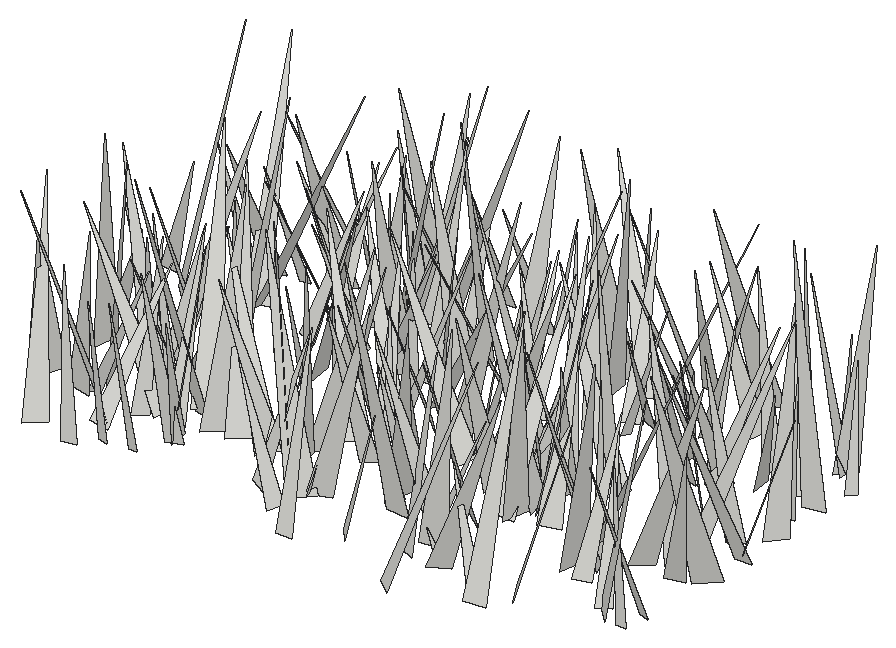
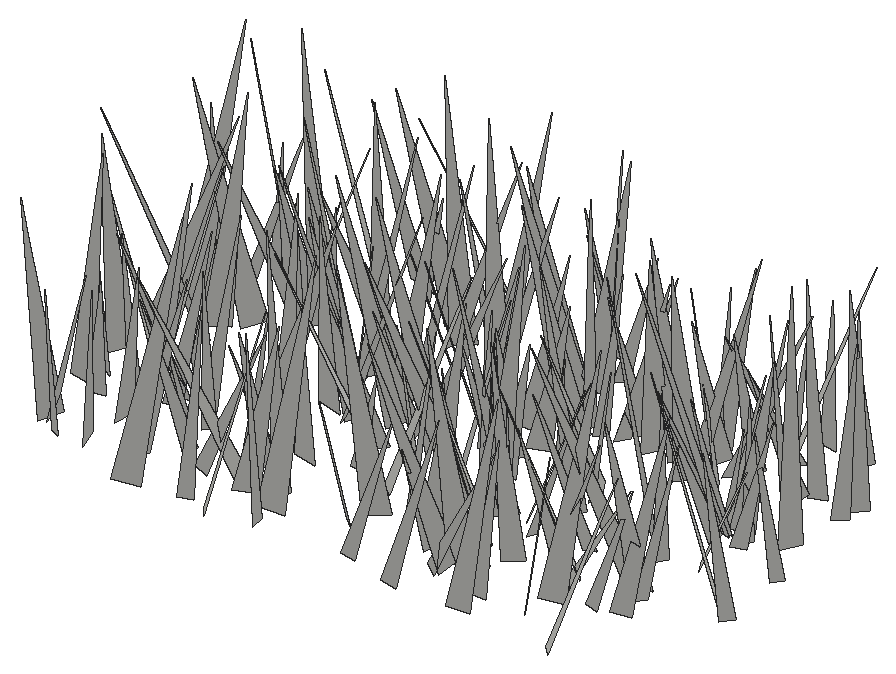
# SketchUp Ruby script. Lengths in inches.
U = 1.inch
M = Sketchup.active_model
def pt(a) = Geom::Point3d.new(a.map { |v| v * U })
def face(e, loops, mat)
  f = e.add_face(loops[0].map { |a| pt(a) })
  loops[1..].each { |l| e.add_face(l.map { |a| pt(a) }).erase! }
  f.material = f.back_material = mat if mat
  f
end
# faces: each face lists its corners as indices into pts; further lists are holes
def faces(e, pts, list, mat = nil) = list.each { |f| face(e, (f[0].is_a?(Array) ? f : [f]).map { |l| l.map { |i| pts[i] } }, mat) }
# xy, xz, yz: faces in a plane at the given z, y or x. An outline is a flat list of corners, or four numbers for a rectangle; further outlines are holes
def ring(l) = l.size == 4 ? [[l[0], l[1]], [l[2], l[1]], [l[2], l[3]], [l[0], l[3]]] : l.each_slice(2).to_a
def flat(e, list, mat, &to3) = list.each { |f| face(e, (f[0].is_a?(Array) ? f : [f]).map { |l| ring(l).map { |u, v| to3.(u, v) } }, mat) }
def xy(e, z, list, mat = nil) = flat(e, list, mat) { |x, y| [x, y, z] }
def xz(e, y, list, mat = nil) = flat(e, list, mat) { |x, z| [x, y, z] }
def yz(e, x, list, mat = nil) = flat(e, list, mat) { |y, z| [x, y, z] }
def lines(e, pts, list) = list.each { |a, b| e.add_line(pt(pts[a]), pt(pts[b])) }
# prism: a flat outline (further loops are holes) pulled along v
def prism(e, loops, v, mat = nil)
  f = face(e, loops, mat); d = Geom::Vector3d.new(v.map { |x| x * U })
  f.pushpull(f.normal.samedirection?(d) ? d.length : -d.length)
end
def box(e, o, s, mat = nil) = prism(e, [[o, [o[0] + s[0], o[1], o[2]], [o[0] + s[0], o[1] + s[1], o[2]], [o[0], o[1] + s[1], o[2]]]], [0, 0, s[2]], mat)
def at(x, y, z, deg = 0) = Geom::Transformation.translation(pt([x, y, z])) * Geom::Transformation.rotation(ORIGIN, Z_AXIS, deg.degrees)
def axes(o, x, y, z) = Geom::Transformation.new([*x, 0, *y, 0, *z, 0, *pt(o).to_a, 1])
def part(name) = M.definitions.add(name)
# library, detail: a bought-in or finely detailed component or shape, given as its bounding box
def library(name, o, s) = part(name).tap { |d| box(d.entities, o, s) }
def detail(e, o, s) = box(e.add_group.entities, o, s)
def put(e, d, t, mat = nil) = e.add_instance(d, t).tap { |i| i.material = mat if mat }
def group(e, t, mat = nil) = e.add_group.tap { |g| g.transformation = t; g.material = mat if mat }.entities
root = M.entities
c1 = part("fur_instance\#9")
p = [[0.8125,0,1.79],[0.67,-0.02,1.48],[0,-0.11,0],[0,0.11,0]]
faces(c1.entities,p,[[0,1,2,3]])
put(root,c1,axes([511.91,80.5,-21.66],[-0.00345,4.9845,1.60202],[5.18158,-0.22632,0.71534],[-0.75028,-1.58596,4.93291]))
put(root,c1,axes([535.35,78.69,-21.66],[4.61833,5.37447,0.17353],[5.34108,-4.61135,0.67253],[-0.62281,0.30742,7.05419]))
put(root,c1,axes([527.52,79.72,-21.66],[0.92539,5.82013,0.73982],[5.78512,-1.02986,0.86568],[-0.97656,-0.58571,5.82931]))
put(root,c1,axes([530.06,81.87,-21.66],[3.37975,2.64749,1.02841],[2.82915,-3.2791,-0.85611],[-0.25046,-1.31446,4.20701]))
put(root,c1,axes([539.36,81.6,-21.66],[-2.08975,2.94897,0.92989],[3.09202,1.98432,0.65582],[-0.0238,-1.13764,3.55435]))
put(root,c1,axes([525.2,81.91,-21.66],[-3.9914,1.89648,0.82188],[2.01712,3.964,0.64912],[0.45094,-0.94526,4.3711]))
put(root,c1,axes([536.39,82.21,-21.66],[5.35038,-4.23141,0.69897],[-4.27634,-5.17862,1.38378],[0.32603,1.51562,6.67957]))
put(root,c1,axes([513.27,81.77,-21.66],[-1.82115,-3.36265,1.61921],[-3.73204,1.65736,-0.7556],[0.03439,1.7865,3.74875]))
put(root,c1,axes([515.16,82,-21.66],[-1.86227,-3.58892,1.59018],[-3.91628,1.57852,-1.02377],[-0.26793,1.87217,3.91156]))
put(root,c1,axes([541.4375,82.52,-21.66],[5.88028,2.97965,0.94292],[3.11911,-5.72141,-1.37172],[-0.19635,-1.65292,6.44782]))
put(root,c1,axes([511.94,83.89,-21.66],[-5.99234,-4.15881,0.58341],[-4.19764,5.96205,-0.6148],[0.12593,0.83815,7.26814]))
put(root,c1,axes([509.05,81.12,-21.66],[-5.83364,4.02968,1.05878],[3.90844,5.92385,-1.01134],[1.44341,0.24573,7.01761]))
put(root,c1,axes([534.62,83.93,-21.66],[2.7668,-7.06079,2.0724],[-7.35623,-2.5972,0.97226],[0.18857,2.28135,7.52095]))
put(root,c1,axes([516.43,84.03,-21.66],[0.40641,-5.35004,1.66525],[-5.54368,-0.62666,-0.66032],[-0.81458,1.59547,5.32467]))
put(root,c1,axes([516.32,84.54,-21.66],[4.42301,-0.66017,1.25029],[-0.31732,-4.46498,-1.23502],[-1.37781,-1.09094,4.29808]))
put(root,c1,axes([540.4,80.28,-21.66],[0.71123,8.26754,0.30404],[8.18462,-0.74766,1.1847],[-1.20692,-0.19821,8.21307]))
put(root,c1,axes([523.04,83.15,-21.66],[2.00403,4.77087,1.2081],[4.88814,-1.77806,-1.08691],[0.57161,-1.52123,5.05925]))
put(root,c1,axes([534.01,82.375,-21.66],[2.59525,5.12132,1.23508],[5.09738,-2.78884,0.85303],[-1.33041,-0.69505,5.67763]))
put(root,c1,axes([506.05,85.07,-21.66],[5.02867,-2.50397,0.95955],[-2.41233,-5.11484,-0.70513],[-1.17101,-0.21602,5.57317]))
put(root,c1,axes([534.87,84.39,-21.66],[-6.53044,0.59698,0.86107],[0.69842,6.53195,0.76827],[0.78105,-0.84949,6.51251]))
put(root,c1,axes([525.59,83.6875,-21.66],[-4.55755,6.1935,2.40469],[6.62517,4.45559,1.08074],[0.49905,-2.58872,7.61332]))
put(root,c1,axes([524.87,83.6,-21.66],[-5.85102,-5.01294,3.05498],[-5.59861,6.06235,-0.77491],[1.76582,2.61061,7.66574]))
put(root,c1,axes([546.52,83.84,-21.66],[-3.91032,-4.73518,3.93684],[-5.20514,5.03349,0.88414],[3.29046,2.33522,6.07707]))
put(root,c1,axes([548.22,83.29,-21.66],[0.93593,4.40998,1.37185],[4.37962,-1.29175,1.16453],[-1.46587,-1.0437,4.3552]))
put(root,c1,axes([548.48,84.95,-21.66],[-2.25031,-4.2676,0.76277],[-4.32128,2.13921,-0.77999],[-0.34742,1.03417,4.76108]))
put(root,c1,axes([508.67,85.4,-21.66],[0.4901,-6.09421,1.40714],[-6.12992,-0.18765,1.32232],[1.24239,1.47818,5.96918]))
put(root,c1,axes([530.84,85.52,-21.66],[-1.51779,-7.89387,2.17922],[-8.18213,1.37007,-0.73587],[-0.33897,2.275,8.00471]))
put(root,c1,axes([526.27,84.42,-21.66],[4.89354,-4.52263,1.72188],[-4.82903,-4.72322,1.31813],[-0.31551,2.14541,6.53173]))
put(root,c1,axes([529.74,87.01,-21.66],[6.8807,-3.2851,0.24825],[-3.20439,-6.80705,-1.26238],[-0.76512,-1.03432,7.51946]))
put(root,c1,axes([511.95,83.04,-21.66],[-0.74484,5.04348,0.31723],[4.84937,0.80355,-1.38926],[1.42161,-0.09859,4.90524]))
put(root,c1,axes([506.35,86.375,-21.66],[4.04472,-2.80495,1.23292],[-2.68281,-4.22845,-0.81868],[-1.47998,-0.00072,4.85358]))
put(root,c1,axes([525.9,84.68,-21.66],[7.69259,-0.4984,1.40276],[-0.64413,-7.77059,0.77146],[-1.3421,0.87272,7.67002]))
put(root,c1,axes([541.98,87,-21.66],[7.73764,-3.02475,0.93063],[-2.93122,-7.77665,-0.90436],[-1.19293,-0.51074,8.25847]))
put(root,c1,axes([534.57,87.54,-21.66],[-3.08937,-5.14938,0.76665],[-5.09175,3.1744,0.80332],[1.08532,0.23487,5.95105]))
put(root,c1,axes([522.34,87.27,-21.66],[3.93846,-2.19121,0.70559],[-1.95473,-3.92185,-1.26841],[-1.21585,-0.79274,4.32481]))
put(root,c1,axes([529.62,87.15,-21.66],[-2.67742,-5.68655,1.10676],[-5.79247,2.6077,-0.61446],[-0.09527,1.2623,6.25523]))
put(root,c1,axes([546.22,84.32,-21.66],[-4.08982,2.78235,0.32679],[2.66533,4.04258,-1.06229],[0.86271,0.7007,4.83111]))
put(root,c1,axes([513.89,86.34,-21.66],[-6.12139,2.10353,0.29479],[2.12072,6.0019,1.20952],[-0.1196,-1.23917,6.35872]))
put(root,c1,axes([521.13,86.87,-21.66],[-5.2528,1.04607,1.18822],[1.28573,5.22141,1.0871],[0.92359,-1.31932,5.24446]))
put(root,c1,axes([523.26,87.07,-21.66],[6.36794,0.62079,2.33056],[0.97414,-6.68136,-0.88201],[-2.20634,-1.15823,6.33704]))
put(root,c1,axes([513.05,85.3,-21.66],[-4.28711,2.60894,1.39768],[2.40918,4.50508,-1.01958],[1.71929,0.19268,4.91389]))
put(root,c1,axes([509.375,85.92,-21.66],[3.95352,-1.35205,0.74696],[-1.51739,-3.78343,1.18299],[-0.28899,1.3689,4.00736]))
put(root,c1,axes([515.64,87.48,-21.66],[-3.53449,-6.31522,1.62159],[-6.50822,3.306,-1.31053],[-0.39309,2.04757,7.11738]))
put(root,c1,axes([533,86.78,-21.66],[2.4928,2.63766,0.46244],[2.65596,-2.35455,-0.88721],[0.34203,-0.94022,3.51911]))
put(root,c1,axes([542.6,88.11,-21.66],[-3.61548,-1.81279,0.7212],[-1.71327,3.67656,0.65243],[0.9333,-0.2734,3.99152]))
put(root,c1,axes([529.875,87.75,-21.66],[0.54062,-3.9189,1.26852],[-4.01221,-0.79056,-0.73238],[-0.93225,1.12979,3.88763]))
put(root,c1,axes([515.33,85.42,-21.66],[-4.48164,3.41054,1.04148],[3.17852,4.57879,-1.31654],[1.61662,0.45221,5.47573]))
put(root,c1,axes([543.35,85.97,-21.66],[-2.74828,4.07366,1.32335],[3.94461,3.01992,-1.10419],[1.66916,-0.42944,4.78838]))
put(root,c1,axes([521.12,86.36,-21.66],[-5.13567,3.95215,0.39173],[3.97037,5.09374,0.66187],[-0.09557,-0.76314,6.44644]))
put(root,c1,axes([513.79,87.8,-21.66],[4.93042,2.67254,1.54888],[2.99605,-4.84755,-1.1728],[-0.75178,-1.79146,5.48417]))
put(root,c1,axes([543.22,87.61,-21.66],[-5.70122,-3.26457,0.62497],[-3.32356,5.6155,-0.98593],[0.04408,1.16649,6.49533]))
put(root,c1,axes([548.85,90.1,-21.66],[4.03591,-7.21522,0.98619],[-7.10178,-4.1491,-1.2924],[-1.61145,0.21471,8.16564]))
put(root,c1,axes([547.27,89.19,-21.66],[2.80299,-5.03768,0.10257],[-5.00094,-2.76705,0.76127],[0.6159,0.45904,5.71449]))
put(root,c1,axes([517.29,86.46,-21.66],[5.828,-3.21448,3.45143],[-4.0564,-6.21538,1.06086],[-2.40642,2.69201,6.57061]))
put(root,c1,axes([526.02,89.09,-21.66],[1.56838,-4.91392,1.31708],[-4.91027,-1.82266,-0.95305],[-1.33063,0.93404,5.06933]))
put(root,c1,axes([509.39,87.3,-21.66],[-5.60874,-1.91132,2.91151],[-2.48414,6.06379,-0.80475],[2.44113,1.77916,5.87056]))
put(root,c1,axes([536.06,89.32,-21.66],[7.26083,-2.43104,1.92439],[-2.31077,-7.51014,-0.76873],[-2.06726,-0.14373,7.61831]))
put(root,c1,axes([523.2,88.29,-21.66],[5.70203,-3.94241,1.833],[-4.2894,-5.59456,1.31056],[-0.70959,2.13867,6.80721]))
put(root,c1,axes([518.92,86.71,-21.66],[5.10712,-2.96498,5.20518],[-4.57955,-6.3419,0.88079],[-3.86171,3.59957,5.83935]))
put(root,c1,axes([544.84,89.36,-21.66],[6.03076,-3.95506,0.64167],[-4.00583,-5.92637,1.12057],[0.08689,1.28836,7.12438]))
put(root,c1,axes([533.49,90.86,-21.66],[3.60817,-5.34608,1.25489],[-5.24687,-3.79935,-1.09972],[-1.62036,0.39817,6.35531]))
put(root,c1,axes([510.59,91.06,-21.66],[-2.24525,-3.81491,0.32062],[-3.67914,2.25292,1.04201],[1.05843,-0.26136,4.3022]))
put(root,c1,axes([506.52,90.52,-21.66],[7.00851,-2.19777,2.01204],[-2.01969,-7.2848,-0.92211],[-2.19075,-0.31499,7.28692]))
put(root,c1,axes([542.125,88.31,-21.66],[6.26365,0.83218,0.34032],[0.77044,-6.2027,0.98722],[-0.46342,0.93576,6.24109]))
put(root,c1,axes([542.62,88.38,-21.66],[-4.924,0.48292,1.1816],[0.20052,4.94285,-1.18453],[1.26062,1.10005,4.80373]))
put(root,c1,axes([536.34,90.93,-21.66],[-7.391,-1.41623,2.02124],[-1.14457,7.62073,1.15434],[2.18657,-0.79801,7.4364]))
put(root,c1,axes([515.51,88.07,-21.66],[-5.56313,6.05819,1.00831],[6.02083,5.64819,-0.71719],[1.2116,-0.25113,8.19364]))
put(root,c1,axes([546.35,90.84,-21.66],[-5.45216,4.70878,2.71596],[5.23215,5.58914,0.81316],[1.47433,-2.42158,7.15803]))
put(root,c1,axes([512.55,90.03,-21.66],[3.9235,0.14114,0.37721],[0.06723,-3.8717,0.74932],[-0.3971,0.73898,3.85386]))
put(root,c1,axes([508.625,91.59,-21.66],[3.85883,-1.0172,1.02296],[-0.87371,-3.97244,-0.65425],[-1.14794,-0.39587,3.93665]))
put(root,c1,axes([526.52,92.33,-21.66],[-0.43336,-3.79274,0.22877],[-3.61563,0.48241,1.14868],[1.16807,0.08612,3.64049]))
put(root,c1,axes([536.4,90.9375,-21.66],[7.04246,3.4796,1.7186],[3.70112,-7.09298,-0.80545],[-1.16744,-1.49647,7.81378]))
put(root,c1,axes([509.68,90.77,-21.66],[-3.34146,5.15286,1.47209],[5.35695,3.16362,1.08579],[-0.14849,-1.82317,6.0447]))
put(root,c1,axes([535.42,88.79,-21.66],[-1.59566,7.05244,0.57454],[6.94745,1.67322,-1.24356],[1.34162,-0.27674,7.12297]))
put(root,c1,axes([548.9,93.13,-21.66],[-1.75901,-6.72397,0.92553],[-6.70142,1.56883,-1.33876],[-1.07676,1.22044,6.82009]))
put(root,c1,axes([510.99,90.44,-21.66],[-4.31173,0.11749,0.33288],[0.02447,4.16916,-1.1546],[0.35215,1.14887,4.15592]))
put(root,c1,axes([536.8,93.06,-21.66],[4.83805,-1.95602,0.87332],[-1.75837,-4.85831,-1.14034],[-1.22345,-0.75248,5.09238]))
put(root,c1,axes([522.14,91.13,-21.66],[-3.8319,-0.08961,1.0116],[-0.27638,3.8917,-0.7022],[0.97723,0.7493,3.76807]))
put(root,c1,axes([524.01,90.57,-21.66],[-3.78417,5.30239,0.2634],[5.25954,3.70033,1.07214],[-0.72248,-0.83479,6.42541]))
put(root,c1,axes([510.1875,91.625,-21.66],[0.83525,-3.69964,2.10924],[-4.22949,-0.46947,0.8514],[0.49764,2.21949,3.69595]))
put(root,c1,axes([508.67,92.35,-21.66],[-2.76713,3.18046,1.2921],[3.43249,2.58898,0.97827],[0.05304,-1.61979,4.10065]))
put(root,c1,axes([534.81,93.26,-21.66],[3.60771,1.96245,2.32029],[2.67745,-3.75626,-0.98607],[-1.43745,-2.07119,3.98679]))
put(root,c1,axes([518.16,93.26,-21.66],[-3.2792,-1.26365,1.37089],[-0.97388,3.52607,0.9207],[1.58988,-0.44645,3.3915]))
put(root,c1,axes([530.21,92.37,-21.66],[-6.66331,2.16551,0.21128],[2.17487,6.60915,0.85019],[-0.06344,-0.87375,6.95459]))
put(root,c1,axes([526.24,94.41,-21.66],[-3.04266,-3.74721,0.50143],[-3.60797,3.07034,1.05183],[1.12942,-0.28668,4.71094]))
put(root,c1,axes([538.24,89.52,-21.66],[0.0768,8.17284,0.16546],[8.06568,-0.10268,1.32775],[-1.3295,-0.15078,8.06464]))
put(root,c1,axes([510.43,91.55,-21.66],[4.03025,7.20792,1.49357],[7.34455,-3.82368,-1.36555],[0.49235,-1.96292,8.14446]))
put(root,c1,axes([504.72,93.9,-21.66],[1.3305,-3.93215,0.09517],[-3.71952,-1.22514,1.38031],[1.27907,0.52755,3.91494]))
put(root,c1,axes([531.71,93.16,-21.66],[6.48225,-3.39085,0.68777],[-3.4557,-6.41712,0.9323],[-0.17042,1.14593,7.25591]))
put(root,c1,axes([525.15,91.87,-21.66],[-0.19051,3.61425,0.52762],[3.57644,0.0773,0.76192],[-0.74175,-0.55561,3.53816]))
put(root,c1,axes([534.33,93.01,-21.66],[1.01992,4.1189,1.46608],[4.23417,-0.55549,-1.38501],[1.0893,-1.69737,4.0109]))
put(root,c1,axes([510.3,92.34,-21.66],[3.86814,-0.78573,1.02615],[-1.07279,-3.75781,1.16655],[-0.72076,1.37634,3.77081]))
put(root,c1,axes([546.43,94.87,-21.66],[-4.48519,-3.52054,0.94744],[-3.42145,4.58335,0.83384],[1.25916,-0.08621,5.64055]))
put(root,c1,axes([518.52,91.83,-21.66],[4.75922,3.00167,0.77273],[2.8511,-4.79497,1.06623],[-1.21588,0.50555,5.5248]))
put(root,c1,axes([517.86,94.88,-21.66],[6.9866,-0.46387,0.39437],[-0.38095,-6.874,-1.33651],[-0.47495,-1.31005,6.87325]))
put(root,c1,axes([524.48,92.24,-21.66],[-3.96377,3.38106,0.80717],[3.27975,4.04327,-0.83051],[1.15166,0.12228,5.14327]))
put(root,c1,axes([533.98,94.07,-21.66],[4.85202,-3.37562,1.03104],[-3.52041,-4.75453,1.00059],[-0.25408,1.41409,5.82544]))
put(root,c1,axes([546.23,92.13,-21.66],[3.64323,6.95762,0.66244],[6.95502,-3.53547,-1.11744],[0.68929,-1.10109,7.77386]))
put(root,c1,axes([548.1,94.33,-21.66],[4.88732,1.92922,0.49219],[1.99044,-4.76555,-1.08522],[-0.04774,-1.19066,5.14102]))
put(root,c1,axes([524.73,93.625,-21.66],[4.20289,4.66758,0.96744],[4.74909,-3.98911,-1.38552],[0.41036,-1.63927,6.12625]))
put(root,c1,axes([534.64,92.57,-21.66],[3.51205,7.24819,1.1392],[7.33442,-3.43356,-0.76524],[0.20101,-1.35755,8.01781]))
put(root,c1,axes([534.61,93.95,-21.66],[-7.94923,-1.56442,0.5472],[-1.62855,7.87073,-1.15603],[0.30767,1.24144,8.0188]))
put(root,c1,axes([547.24,94.54,-21.66],[0.3865,-5.10308,2.42648],[-5.49086,-0.91339,-1.04632],[-1.33405,2.28099,5.00959]))
put(root,c1,axes([529.2,94.98,-21.66],[3.2608,1.42212,0.87051],[1.60342,-3.19897,-0.78016],[-0.45742,-1.07574,3.47082]))
put(root,c1,axes([530.23,93.41,-21.66],[4.26964,0.47793,1.18834],[0.14194,-4.28676,1.21405],[-1.27296,1.12502,4.1212]))
put(root,c1,axes([528.43,93.75,-21.66],[7.3545,-2.24014,2.18394],[-2.66673,-7.40612,1.38362],[-1.63595,2.00191,7.56257]))
put(root,c1,axes([538.65,94.53,-21.66],[-1.16984,-6.03511,2.92768],[-6.70455,0.96018,-0.69968],[-0.2073,3.00298,6.1075]))
put(root,c1,axes([538.87,94.71,-21.66],[-5.22041,4.31379,0.87725],[4.39805,5.05275,1.32586],[-0.18846,-1.57859,6.64105]))
put(root,c1,axes([512.71,94.58,-21.66],[4.94057,6.27292,2.28459],[6.62263,-4.9638,-0.69253],[-0.84236,-2.23369,7.95482]))
put(root,c1,axes([511.12,96.125,-21.66],[4.3252,-1.84495,1.08949],[-1.74272,-4.45705,-0.62914],[-1.2465,-0.1704,4.65998]))
put(root,c1,axes([523.49,94.23,-21.66],[-3.54308,4.52564,0.44169],[4.5332,3.47169,0.79207],[-0.35583,-0.83417,5.69276]))
put(root,c1,axes([544.8,94.85,-21.66],[-3.71707,-2.68533,1.32909],[-2.9797,3.53518,-1.19076],[0.31439,1.75658,4.42828]))
put(root,c1,axes([509.03,95.22,-21.66],[-3.56795,-1.90054,0.20659],[-1.88749,3.43261,-1.0196],[-0.30353,0.99505,3.91187]))
put(root,c1,axes([535.87,94.08,-21.66],[0.42916,7.00561,1.64499],[7.11073,-0.66598,0.98114],[-1.10544,-1.56418,6.94983]))
put(root,c1,axes([521.37,97.88,-21.66],[4.41778,-6.32124,1.65754],[-6.32459,-4.6393,-0.83587],[-1.6447,0.86086,7.66656]))
put(root,c1,axes([540.92,98.27,-21.66],[-0.50575,-5.47671,0.42869],[-5.44927,0.55465,0.65709],[0.69543,0.36321,5.46062]))
put(root,c1,axes([527.65,99.33,-21.66],[-3.98509,-5.15803,0.00595],[-5.07141,3.91953,1.18509],[0.94137,-0.71992,6.40951]))
put(root,c1,axes([519.8,96.65,-21.66],[-5.05494,-2.22544,0.30278],[-2.23904,4.935,-1.10864],[-0.17591,1.1357,5.41072]))
put(root,c1,axes([525.05,96.32,-21.66],[6.85637,-0.90607,0.05149],[-0.90407,-6.7849,0.99057],[0.07926,0.98874,6.84468]))
put(root,c1,axes([548.83,96.13,-21.66],[5.64429,-3.09602,3.33103],[-3.78051,-6.14532,0.69416],[-2.52761,2.27789,6.40012]))
put(root,c1,axes([520.56,97.41,-21.66],[4.45339,-2.56263,0.11815],[-2.55046,-4.39735,0.75645],[0.27609,0.71411,5.08208]))
put(root,c1,axes([518.36,98.26,-21.66],[-4.47409,-0.55232,0.95951],[-0.288,4.43762,1.21151],[1.069,-1.11608,4.34221]))
put(root,c1,axes([521.87,98.32,-21.66],[-2.90046,-3.39812,1.38689],[-3.27993,3.19309,0.96417],[1.64705,0.37459,4.36237]))
put(root,c1,axes([523.17,96.41,-21.66],[-4.45117,0.87592,1.04433],[0.68712,4.52233,-0.86441],[1.17717,0.67238,4.45342]))
put(root,c1,axes([542.72,99.22,-21.66],[2.25117,-4.50739,0.41367],[-4.42833,-2.28883,-0.84056],[-0.93676,-0.01195,4.96767]))
put(root,c1,axes([530.92,95.87,-21.66],[-2.87102,4.68172,0.40163],[4.57171,2.89185,-1.02921],[1.08596,0.20316,5.39463]))
put(root,c1,axes([504.1,99.02,-21.66],[1.4923,-4.43759,0.64343],[-4.35505,-1.27294,1.3215],[1.06759,1.01025,4.49142]))
put(root,c1,axes([521.22,96.67,-21.66],[7.46967,2.68884,2.29218],[2.3982,-7.79505,1.32883],[-2.59473,0.53597,7.82688]))
put(root,c1,axes([514.8,97.63,-21.66],[0.90877,4.85728,1.17196],[4.86719,-0.59112,-1.32422],[1.13009,-1.36012,4.76083]))
put(root,c1,axes([539.5,100.01,-21.66],[4.03439,-1.67825,0.01541],[-1.64329,-3.95818,-0.85174],[-0.3411,-0.78061,4.28572]))
put(root,c1,axes([544.43,100.27,-21.66],[4.66467,-0.77947,0.02704],[-0.7406,-4.47818,-1.32848],[-0.24456,-1.30606,4.53893]))
put(root,c1,axes([522.87,99.39,-21.66],[4.02483,1.17033,1.17041],[1.40502,-4.04247,-0.78939],[-0.87491,-1.10794,4.11653]))
put(root,c1,axes([542.56,98.21,-21.66],[2.02103,5.13059,0.73898],[5.12624,-1.86067,-1.10143],[0.76856,-1.08099,5.40318]))
put(root,c1,axes([547.98,98.44,-21.66],[1.43677,3.63281,1.03111],[3.57622,-1.66329,0.8769],[-1.21291,-0.60083,3.80693]))
put(root,c1,axes([523.82,99.97,-21.66],[4.51203,-4.20905,2.90182],[-4.30887,-5.21386,-0.8628],[-2.75143,1.26279,6.10984]))
put(root,c1,axes([509.2,100.24,-21.66],[-4.57691,0.82768,1.57562],[1.18388,4.66198,0.99001],[1.32893,-1.30255,4.54457]))
put(root,c1,axes([530.36,98.45,-21.66],[-1.14245,4.14217,0.46464],[4.01441,0.96381,1.27839],[-1.12161,-0.76952,4.10226]))
put(root,c1,axes([530.07,97.14,-21.66],[5.64336,5.1887,0.30355],[5.15395,-5.64438,0.66329],[-0.67191,0.28398,7.63742]))
put(root,c1,axes([506.14,97.42,-21.66],[-5.10797,-4.03263,5.02727],[-5.71036,5.80586,-1.14484],[2.98787,4.202,6.40647]))
put(root,c1,axes([519.36,98.9375,-21.66],[-4.01098,-1.65554,1.8183],[-2.11594,4.09606,-0.93811],[1.25294,1.61753,4.23659]))
put(root,c1,axes([509.04,102.12,-21.66],[1.9027,-5.40071,0.1352],[-5.35593,-1.9045,-0.70218],[-0.70705,-0.10684,5.68285]))
put(root,c1,axes([535.49,101.78,-21.66],[-0.82646,-4.24361,0.01629],[-4.06802,0.79698,1.2278],[1.20816,-0.21938,4.14533]))
put(root,c1,axes([519.57,101.13,-21.66],[4.8829,2.83209,2.83107],[3.60518,-5.05239,-1.16384],[-1.7431,-2.51617,5.52349]))
put(root,c1,axes([510.49,99.07,-21.66],[7.61599,0.93725,0.32253],[0.89381,-7.57423,0.90437],[-0.42844,0.85927,7.61996]))
put(root,c1,axes([523.23,97.89,-21.66],[1.19903,6.87384,0.5978],[6.78552,-1.2847,1.16229],[-1.25048,-0.38022,6.88014]))
put(root,c1,axes([517.38,101.08,-21.66],[3.13574,-5.33007,1.5739],[-5.55752,-3.01682,0.85589],[-0.02918,1.79133,6.12454]))
put(root,c1,axes([548.32,100.04,-21.66],[-0.94907,-6.99906,3.73248],[-7.88487,0.42284,-1.21201],[-0.8643,3.82797,6.95835]))
put(root,c1,axes([527.21,100.73,-21.66],[1.77196,3.84512,1.4323],[4.08534,-1.50774,-1.0065],[0.38272,-1.70823,4.11239]))
put(root,c1,axes([513.53,101.07,-21.66],[-2.7685,-2.84273,0.0732],[-2.6967,2.59213,-1.32656],[-0.90237,0.97511,3.73978]))
put(root,c1,axes([512.94,103.33,-21.66],[2.89826,-6.60565,0.55734],[-6.55377,-2.94663,-0.84295],[-0.99662,0.16719,7.16407]))
put(root,c1,axes([513.47,100.2,-21.66],[4.56915,3.9518,0.34933],[3.96081,-4.51383,-0.74378],[0.22516,-0.79028,5.99505]))
put(root,c1,axes([533.29,99.43,-21.66],[-0.40472,6.25604,0.83945],[6.18781,0.22712,1.29072],[-1.24649,-0.90382,6.13481]))
put(root,c1,axes([535.0625,100.18,-21.66],[3.77133,0.16267,0.95437],[-0.10228,-3.74984,1.04331],[-0.96272,1.03561,3.6278]))
put(root,c1,axes([514.96,99.92,-21.66],[-0.69382,4.82103,0.91338],[4.82167,0.84094,-0.77604],[0.90996,-0.78004,4.80848]))
put(root,c1,axes([514.3125,102,-21.66],[-4.64353,0.24048,0.81476],[0.40253,4.60984,0.93348],[0.74809,-0.98772,4.55508]))
put(root,c1,axes([541.4375,99.6,-21.66],[1.45734,4.18221,0.34787],[4.02467,-1.49715,1.13854],[-1.18907,0.05834,4.28]))
put(root,c1,axes([510.81,102.5,-21.66],[-0.75955,-3.70224,0.74684],[-3.72635,0.61048,-0.76351],[-0.61539,0.87293,3.70143]))
put(root,c1,axes([510.29,98.94,-21.66],[-0.64935,7.68845,0.01437],[7.6155,0.6412,1.06165],[-1.05669,-0.10353,7.64243]))
put(root,c1,axes([546.79,100.77,-21.66],[-1.86757,4.60063,0.33127],[4.58089,1.80817,0.71369],[-0.53944,-0.57279,4.91369]))
put(root,c1,axes([524.35,101.53,-21.66],[-6.69372,-1.63538,1.73187],[-1.91789,6.76382,-1.02573],[1.41263,1.43387,6.81383]))
put(root,c1,axes([520.12,99.75,-21.66],[5.47327,5.90798,0.9862],[5.7796,-5.55993,1.23167],[-1.57262,0.12835,7.95889]))
put(root,c1,axes([526.42,101.75,-21.66],[-2.68799,6.56885,2.98447],[6.8694,3.30396,-1.08507],[2.20641,-2.2839,7.01411]))
put(root,c1,axes([518.26,102.15,-21.66],[4.16572,3.95636,0.93283],[4.06431,-4.03236,-1.04767],[0.06588,-1.40123,5.64875]))
put(root,c1,axes([531.66,103.49,-21.66],[7.52805,-0.18805,1.99939],[0.07054,-7.72753,-0.99239],[-2.00698,-0.97696,7.46472]))
put(root,c1,axes([543.89,101.93,-21.66],[-5.59826,1.4556,0.99849],[1.35798,5.67289,-0.65612],[1.12768,0.39476,5.74707]))
put(root,c1,axes([537,103.88,-21.66],[-0.83843,-4.56243,0.7415],[-4.45874,0.59959,-1.35228],[-1.2187,0.94513,4.43735]))
put(root,c1,axes([534.55,101.38,-21.66],[-3.134,4.47853,0.59876],[4.43295,3.18866,-0.64743],[0.8745,-0.1137,5.42771]))
put(root,c1,axes([519.28,103.16,-21.66],[3.63637,-5.76719,3.12725],[-6.51934,-3.57646,0.98508],[-0.73369,3.19558,6.74635]))
put(root,c1,axes([548.88,102.59,-21.66],[-3.45785,1.40655,0.59459],[1.25916,3.45892,-0.85969],[0.86397,0.58836,3.63264]))
put(root,c1,axes([531.18,105.01,-21.66],[1.42395,-7.42701,2.10024],[-7.62151,-1.69014,-0.80943],[-1.21824,1.89264,7.51884]))
put(root,c1,axes([540.77,104.48,-21.66],[4.1746,-2.61988,2.8232],[-2.37692,-5.02847,-1.15163],[-3.03059,0.33503,4.79215]))
put(root,c1,axes([538.54,102.74,-21.66],[5.15508,0.33774,1.32609],[0.02228,-5.18864,1.23487],[-1.36825,1.188,5.01637]))
put(root,c1,axes([520.3125,104.63,-21.66],[-2.43952,-3.83837,0.4143],[-3.75379,2.24378,-1.31547],[-0.90209,1.04325,4.3536]))
put(root,c1,axes([513.32,105.13,-21.66],[-3.34648,-2.86729,1.25208],[-2.75468,3.56945,0.81158],[1.4835,0.16004,4.33146]))
put(root,c1,axes([527.27,103.22,-21.66],[2.58432,3.47984,0.90101],[3.42396,-2.72089,0.68775],[-1.09434,-0.29537,4.2796]))
put(root,c1,axes([535.36,102.66,-21.66],[6.4283,2.09347,0.22673],[2.03253,-6.35917,1.08941],[-0.55031,0.96716,6.67224]))
put(root,c1,axes([521.74,102.81,-21.66],[-3.54385,2.2292,0.7922],[1.93522,3.55225,-1.33876],[1.36083,0.75365,3.96686]))
put(root,c1,axes([547.19,104.15,-21.66],[-5.62081,-1.07857,0.79033],[-1.22962,5.511,-1.22409],[0.52534,1.35906,5.59093]))
put(root,c1,axes([519.67,103.88,-21.66],[7.1879,-0.3196,1.18159],[-0.53762,-7.14753,1.33717],[-1.09967,1.40532,7.06966]))
put(root,c1,axes([547.17,104.27,-21.66],[-5.57842,3.33095,2.99608],[3.28064,6.29556,-0.89096],[3.05108,-0.67911,6.43585]))
put(root,c1,axes([535.6875,106.85,-21.66],[0.34868,-5.31048,0.36463],[-5.26358,-0.28954,0.81646],[0.79301,0.41316,5.25892]))
put(root,c1,axes([539.31,107.54,-21.66],[2.6009,-7.25193,0.96085],[-7.2129,-2.71231,-0.94648],[-1.21974,0.57558,7.64587]))
put(root,c1,axes([516.49,105.375,-21.66],[0.55696,-4.64877,2.01019],[-4.98122,-0.86859,-0.62855],[-0.91614,1.89648,4.63963]))
put(root,c1,axes([524.76,106.36,-21.66],[0.09538,-4.31944,0.7575],[-4.29634,-0.24392,-0.84995],[-0.8791,0.72346,4.23607]))
put(root,c1,axes([545.83,105.62,-21.66],[-1.72893,-3.46771,1.76985],[-3.62718,2.13831,0.64633],[1.41454,1.24466,3.82053]))
put(root,c1,axes([533.6,104.21,-21.66],[-4.22823,5.63878,0.60494],[5.64653,4.11564,1.10357],[-0.52773,-1.14251,6.96102]))
put(root,c1,axes([534,107.37,-21.66],[-4.57132,-4.01454,0.83204],[-3.89365,4.6413,1.00178],[1.28384,-0.21818,6.00082]))
put(root,c1,axes([509.72,107.77,-21.66],[-3.92471,-3.72483,0.22437],[-3.66233,3.90735,0.80501],[0.71557,-0.43166,5.35067]))
put(root,c1,axes([530.95,106.51,-21.66],[5.21956,1.10973,1.69595],[1.36173,-5.39042,-0.66376],[-1.50115,-1.03121,5.29478]))
put(root,c1,axes([543.97,105.03,-21.66],[-5.50715,-0.70612,1.61288],[-1.08889,5.52799,-1.29784],[1.38358,1.53996,5.39842]))
put(root,c1,axes([516.32,107.26,-21.66],[1.47343,-6.07806,1.78682],[-6.21699,-1.74005,-0.79238],[-1.21846,1.52838,6.20371]))
put(root,c1,axes([521.0625,107.4375,-21.66],[-0.49716,-5.04462,0.80589],[-5.07325,0.39247,-0.67299],[-0.59982,0.86174,5.02418]))
